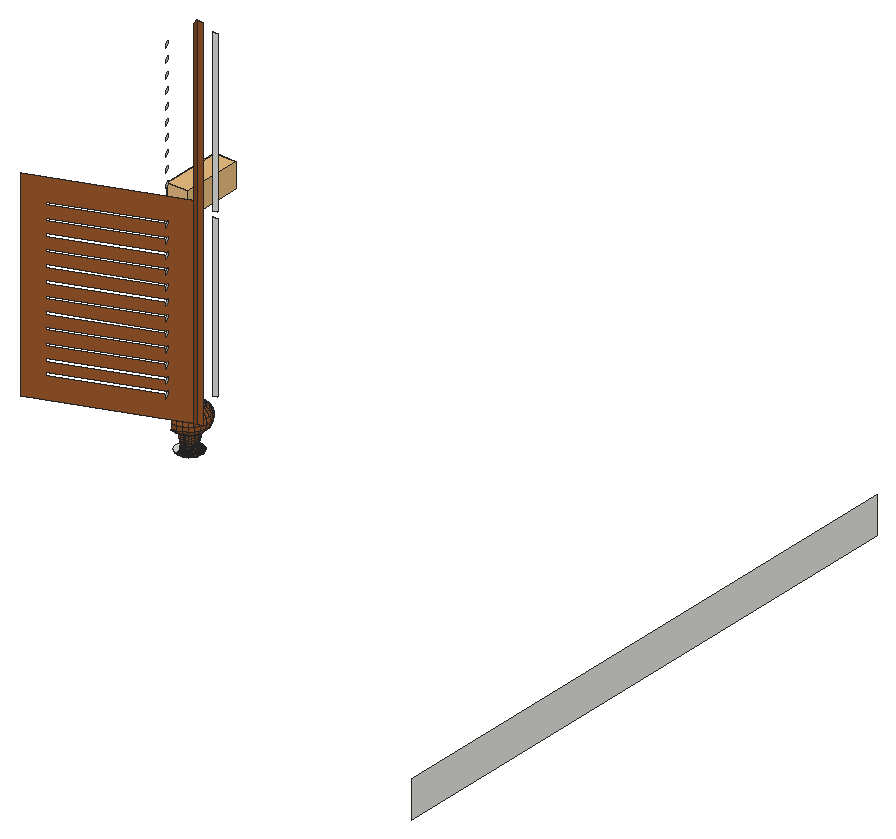
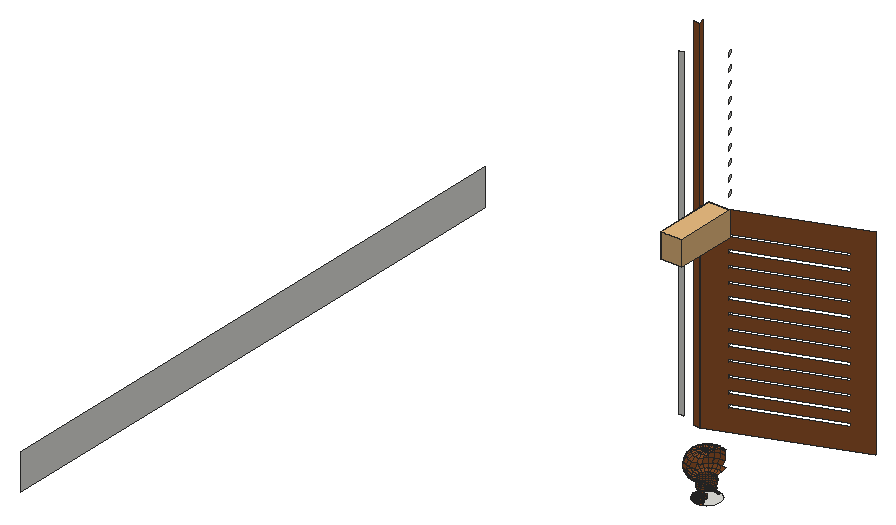
# SketchUp Ruby script. Lengths in inches.
U = 1.inch
M = Sketchup.active_model
def pt(a) = Geom::Point3d.new(a.map { |v| v * U })
def face(e, loops, mat)
  f = e.add_face(loops[0].map { |a| pt(a) })
  loops[1..].each { |l| e.add_face(l.map { |a| pt(a) }).erase! }
  f.material = f.back_material = mat if mat
  f
end
# faces: each face lists its corners as indices into pts; further lists are holes
def faces(e, pts, list, mat = nil) = list.each { |f| face(e, (f[0].is_a?(Array) ? f : [f]).map { |l| l.map { |i| pts[i] } }, mat) }
# xy, xz, yz: faces in a plane at the given z, y or x. An outline is a flat list of corners, or four numbers for a rectangle; further outlines are holes
def ring(l) = l.size == 4 ? [[l[0], l[1]], [l[2], l[1]], [l[2], l[3]], [l[0], l[3]]] : l.each_slice(2).to_a
def flat(e, list, mat, &to3) = list.each { |f| face(e, (f[0].is_a?(Array) ? f : [f]).map { |l| ring(l).map { |u, v| to3.(u, v) } }, mat) }
def xy(e, z, list, mat = nil) = flat(e, list, mat) { |x, y| [x, y, z] }
def xz(e, y, list, mat = nil) = flat(e, list, mat) { |x, z| [x, y, z] }
def yz(e, x, list, mat = nil) = flat(e, list, mat) { |y, z| [x, y, z] }
def lines(e, pts, list) = list.each { |a, b| e.add_line(pt(pts[a]), pt(pts[b])) }
# prism: a flat outline (further loops are holes) pulled along v
def prism(e, loops, v, mat = nil)
  f = face(e, loops, mat); d = Geom::Vector3d.new(v.map { |x| x * U })
  f.pushpull(f.normal.samedirection?(d) ? d.length : -d.length)
end
def box(e, o, s, mat = nil) = prism(e, [[o, [o[0] + s[0], o[1], o[2]], [o[0] + s[0], o[1] + s[1], o[2]], [o[0], o[1] + s[1], o[2]]]], [0, 0, s[2]], mat)
def at(x, y, z, deg = 0) = Geom::Transformation.translation(pt([x, y, z])) * Geom::Transformation.rotation(ORIGIN, Z_AXIS, deg.degrees)
def axes(o, x, y, z) = Geom::Transformation.new([*x, 0, *y, 0, *z, 0, *pt(o).to_a, 1])
def part(name) = M.definitions.add(name)
# library, detail: a bought-in or finely detailed component or shape, given as its bounding box
def library(name, o, s) = part(name).tap { |d| box(d.entities, o, s) }
def detail(e, o, s) = box(e.add_group.entities, o, s)
def put(e, d, t, mat = nil) = e.add_instance(d, t).tap { |i| i.material = mat if mat }
def group(e, t, mat = nil) = e.add_group.tap { |g| g.transformation = t; g.material = mat if mat }.entities
root = M.entities
M.materials.add("[Color M03]").color = [170, 170, 170]
M.materials.add("[Wood Cherry Original]").color = [152, 86, 42]
c1 = library("Group\#10",[0,0,0],[6.05,17.1,6.94])
xy(root,6,[[197.18,47.97,197.74,47.97,198.28,48.11,198.76,48.39,199.16,48.78,199.4375,49.26,199.59,49.8,199.59,50.36,199.44,50.9,199.17,51.38,198.77,51.78,198.29,52.06,197.75,52.21,197.19,52.21,196.65,52.07,196.17,51.79,195.77,51.4,195.49,50.91,195.35,50.375,195.34,49.82,195.49,49.28,195.76,48.79,196.16,48.4,196.64,48.11]])
xy(root,6,[[197.18,47.97,197.2,48.12,196.7,48.25,196.64,48.11],[197.18,47.97,197.74,47.97,197.72,48.12,197.2,48.12],[197.74,47.97,198.28,48.11,198.22,48.25,197.72,48.12],[198.28,48.11,198.76,48.39,198.67,48.51,198.22,48.25],[198.76,48.39,199.16,48.78,199.04,48.87,198.67,48.51],
  [199.16,48.78,199.4375,49.26,199.3,49.32,199.04,48.87],[199.4375,49.26,199.59,49.8,199.44,49.82,199.3,49.32],[199.59,49.8,199.59,50.36,199.4375,50.34,199.44,49.82],[199.4375,50.34,199.59,50.36,199.44,50.9,199.3,50.84],[199.3,50.84,199.44,50.9,199.17,51.38,199.05,51.29],
  [199.05,51.29,199.17,51.38,198.77,51.78,198.68,51.66],[198.68,51.66,198.77,51.78,198.29,52.06,198.23,51.92],[198.23,51.92,198.29,52.06,197.75,52.21,197.73,52.06],[196.71,51.93,197.21,52.06,197.19,52.21,196.65,52.07],[197.21,52.06,197.73,52.06,197.75,52.21,197.19,52.21]],"[Wood Cherry Original]")
xz(root,46.11,[[201.81,13.08,202.9,73.08]],"[Wood Cherry Original]")
xz(root,48.59,[[197.26,8.1,197.66,8.4]],"[Wood Cherry Original]")
xz(root,49.11,[[202.15,16.08,202.9,42.58],[202.15,43.58,202.9,70.08]])
xz(root,51.28,[[197.3125,6.79,197.63,6.94]],"[Wood Cherry Original]")
yz(root,198.66,[[49.93,6.79,50.24,6.94]],"[Wood Cherry Original]")
yz(root,198.96,[[49.88,8.1,50.28,8.4]],"[Wood Cherry Original]")
yz(root,274.48,[[0,0,96.25,6]])
p = [[196.76,48.39,6.03],[196.7,48.25,6],[197.2,48.12,6],[197.22,48.27,6.03],[197.72,48.12,6],[197.7,48.26,6.03],
  [198.22,48.25,6],[198.16,48.39,6.03],[198.67,48.51,6],[198.58,48.625,6.03],[196.81,48.52,6.08],[197.24,48.41,6.08],
  [197.68,48.4,6.08],[198.11,48.52,6.08],[198.49,48.74,6.08],[199.04,48.87,6],[198.92,48.96,6.03],[198.81,49.05,6.08],
  [199.3,49.32,6],[199.16,49.375,6.03],[199.03,49.43,6.08],[199.44,49.82,6],[199.29,49.84,6.03],[199.15,49.86,6.08],
  [199.29,50.32,6.03],[199.15,50.3,6.08],[199.4375,50.34,6],[199.17,50.78,6.03],[199.04,50.73,6.08],[199.3,50.84,6],
  [198.93,51.2,6.03],[198.82,51.11,6.08],[199.05,51.29,6],[198.59,51.54,6.03],[198.5,51.43,6.08],[198.68,51.66,6],
  [198.18,51.78,6.03],[198.12,51.65,6.08],[198.23,51.92,6],[197.25,51.77,6.08],[197.23,51.91,6.03],[196.77,51.79,6.03],
  [196.82,51.66,6.08],[197.71,51.91,6.03],[197.69,51.77,6.08],[197.21,52.06,6],[196.71,51.93,6],[197.73,52.06,6],
  [196.86,48.64,6.16],[197.26,48.54,6.16],[197.66,48.53,6.16],[198.06,48.64,6.16],[198.41,48.84,6.16],[198.7,49.13,6.16],
  [198.91,49.48,6.16],[199.02,49.875,6.16],[199.02,50.29,6.16],[198.91,50.68,6.16],[198.71,51.04,6.16],[198.42,51.33,6.16],
  [198.07,51.53,6.16],[197.27,51.64,6.16],[196.87,51.54,6.16],[197.68,51.64,6.16],[196.91,48.75,6.25],[197.27,48.65,6.25],
  [197.65,48.65,6.25],[198.02,48.74,6.25],[198.34,48.93,6.25],[198.61,49.2,6.25],[198.8,49.53,6.25],[198.9,49.89,6.25],
  [198.9,50.27,6.25],[198.81,50.64,6.25],[198.62,50.97,6.25],[198.35,51.23,6.25],[198.03,51.43,6.25],[197.28,51.53,6.25],
  [196.92,51.43,6.25],[197.66,51.52,6.25],[196.94,48.84,6.37],[197.28,48.75,6.37],[197.64,48.74,6.37],[197.98,48.83,6.37],
  [198.29,49.01,6.37],[198.54,49.26,6.37],[198.71,49.5625,6.37],[198.81,49.91,6.37],[198.81,50.26,6.37],[198.72,50.6,6.37],
  [198.54,50.91,6.37],[198.29,51.16,6.37],[197.99,51.34,6.37],[197.29,51.43,6.37],[196.95,51.34,6.37],[197.65,51.43,6.37],
  [196.97,48.91,6.5],[197.29,48.82,6.5],[197.63,48.82,6.5],[197.95,48.9,6.5],[198.24,49.07,6.5],[198.48,49.3,6.5],
  [198.65,49.59,6.5],[198.73,49.92,6.5],[198.73,50.25,6.5],[198.65,50.57,6.5],[198.48,50.86,6.5],[198.25,51.1,6.5],
  [197.96,51.27,6.5],[197.3,51.36,6.5],[196.98,51.27,6.5],[197.64,51.35,6.5],[196.99,48.95,6.64],[197.3,48.87,6.64],
  [197.62,48.87,6.64],[197.93,48.95,6.64],[196.71,49.12,6.64],[196.68,49.08,6.5],[198.21,49.11,6.64],[198.4375,49.34,6.64],
  [198.6,49.61,6.64],[198.68,49.92,6.64],[198.68,50.24,6.64],[198.6,50.55,6.64],[198.44,50.83,6.64],[198.22,51.06,6.64],
  [197,51.22,6.64],[196.69,51.1,6.5],[196.72,51.0625,6.64],[197.94,51.22,6.64],[197.31,51.3,6.64],[197.63,51.3,6.64],
  [197,48.98,6.79],[197.3,48.9,6.79],[197.62,48.9,6.79],[197.92,48.98,6.79],[196.73,49.14,6.79],[198.19,49.13,6.79],
  [198.42,49.35,6.79],[198.57,49.62,6.79],[198.66,49.93,6.79],[198.66,50.24,6.79],[198.58,50.54,6.79],[198.42,50.82,6.79],
  [198.2,51.04,6.79],[197.01,51.2,6.79],[196.74,51.04,6.79],[197.93,51.2,6.79],[197.3125,51.28,6.79],[197.63,51.28,6.79],
  [197,48.98,6.94],[197.3,48.9,6.94],[197.62,48.89,6.94],[197.92,48.97,6.94],[196.73,49.14,6.94],[198.19,49.13,6.94],
  [198.42,49.35,6.94],[198.57,49.62,6.94],[198.66,49.93,6.94],[198.66,50.24,6.94],[198.58,50.54,6.94],[198.42,50.82,6.94],
  [198.2,51.04,6.94],[197.01,51.2,6.94],[196.74,51.04,6.94],[197.93,51.2,6.94],[197.3125,51.28,6.94],[197.63,51.28,6.94],
  [196.99,48.95,7.09],[197.3,48.87,7.09],[197.62,48.87,7.09],[197.93,48.95,7.09],[196.71,49.12,7.09],[198.21,49.11,7.09],
  [198.4375,49.34,7.09],[198.6,49.61,7.09],[198.68,49.92,7.09],[198.68,50.24,7.09],[198.6,50.55,7.09],[198.44,50.83,7.09],
  [198.22,51.06,7.09],[197,51.22,7.09],[196.72,51.06,7.09],[197.94,51.22,7.09],[197.31,51.31,7.09],[197.63,51.3,7.09],
  [196.97,48.91,7.23],[197.29,48.82,7.23],[197.63,48.82,7.23],[197.95,48.9,7.23],[196.68,49.07,7.23],[198.24,49.07,7.23],
  [198.48,49.3,7.23],[198.65,49.59,7.23],[198.73,49.92,7.23],[198.74,50.25,7.23],[198.65,50.57,7.23],[198.48,50.86,7.23],
  [198.25,51.1,7.23],[196.98,51.27,7.23],[196.69,51.11,7.23],[197.96,51.27,7.23],[197.3,51.36,7.23],[197.64,51.36,7.23],
  [196.93,48.8,7.51],[197.28,48.71,7.51],[197.64,48.71,7.51],[197.99,48.8,7.51],[198.31,48.98,7.51],[198.57,49.24,7.51],
  [198.75,49.55,7.51],[198.84,49.9,7.51],[198.85,50.26,7.51],[198.75,50.61,7.51],[198.57,50.93,7.51],[198.32,51.1875,7.51],
  [198,51.37,7.51],[197.29,51.47,7.51],[196.9375,51.375,7.51],[197.65,51.47,7.51],[196.9,48.73,7.8],[197.27,48.63,7.8],
  [197.65,48.63,7.8],[198.02,48.73,7.8],[198.35,48.92,7.8],[198.625,49.1875,7.8],[198.82,49.52,7.8],[198.92,49.89,7.8],
  [198.92,50.27,7.8],[198.82,50.64,7.8],[198.63,50.98,7.8],[198.36,51.25,7.8],[198.03,51.44,7.8],[197.28,51.54,7.8],
  [196.91,51.45,7.8],[197.66,51.54,7.8],[196.88,48.7,8.1],[197.26,48.59,8.1],[197.66,48.59,8.1],[198.04,48.69,8.1],
  [198.38,48.89,8.1],[198.66,49.16,8.1],[198.86,49.5,8.1],[198.96,49.88,8.1],[198.96,50.28,8.1],[198.86,50.66,8.1],
  [198.66,51,8.1],[198.39,51.28,8.1],[198.05,51.48,8.1],[197.27,51.58,8.1],[196.89,51.48,8.1],[197.67,51.58,8.1],
  [196.88,48.69,8.4],[197.26,48.59,8.4],[197.66,48.59,8.4],[198.04,48.69,8.4],[198.38,48.89,8.4],[198.66,49.16,8.4],
  [198.86,49.5,8.4],[198.96,49.88,8.4],[198.96,50.28,8.4],[198.86,50.66,8.4],[198.67,51,8.4],[198.39,51.28,8.4],
  [198.05,51.48,8.4],[197.27,51.59,8.4],[196.89,51.48,8.4],[197.67,51.58,8.4],[196.9,48.73,8.7],[197.27,48.625,8.7],
  [197.65,48.62,8.7],[198.03,48.72,8.7],[198.36,48.91,8.7],[198.63,49.18,8.7],[198.83,49.52,8.7],[198.93,49.89,8.7],
  [198.93,50.27,8.7],[198.83,50.65,8.7],[198.64,50.98,8.7],[198.37,51.25,8.7],[198.04,51.45,8.7],[197.66,51.55,8.7],
  [197.28,51.55,8.7],[196.91,51.45,8.7],[196.92,48.79,8.99],[197.28,48.69,8.99],[197.64,48.69,8.99],[198,48.79,8.99],
  [198.32,48.97,8.99],[198.58,49.23,8.99],[198.76,49.54,8.99],[198.86,49.9,8.99],[198.86,50.27,8.99],[198.77,50.62,8.99],
  [198.58,50.9375,8.99],[198.33,51.2,8.99],[198.01,51.38,8.99],[197.29,51.48,8.99],[196.93,51.39,8.99],[197.65,51.48,8.99],
  [196.65,48.14,9.21],[197.18,48,9.21],[197.73,48,9.21],[198.26,48.14,9.21],[198.74,48.41,9.21],[199.13,48.8,9.21],
  [199.41,49.27,9.21],[199.55,49.8,9.21],[199.56,50.35,9.21],[199.42,50.89,9.21],[199.14,51.36,9.21],[198.76,51.75,9.21],
  [198.28,52.03,9.21],[197.2,52.18,9.21],[196.67,52.04,9.21],[197.75,52.18,9.21],[196.43,47.61,9.66],[197.1,47.42,9.66],
  [197.81,47.42,9.66],[198.48,47.6,9.66],[199.09,47.95,9.66],[199.59,48.44,9.66],[199.94,49.05,9.66],[200.13,49.73,9.66],
  [200.13,50.43,9.66],[199.95,51.11,9.66],[199.6,51.71,9.66],[199.11,52.21,9.66],[198.5,52.57,9.66],[197.125,52.75,9.66],
  [196.45,52.57,9.66],[197.83,52.75,9.66],[197.05,47.05,10.28],[197.85,47.04,10.28],[198.63,47.25,10.28],[199.32,47.65,10.28],
  [199.89,48.21,10.28],[200.29,48.9,10.28],[200.51,49.68,10.28],[200.51,50.48,10.28],[200.3,51.25,10.28],[199.91,51.94,10.28],
  [199.34,52.51,10.28],[198.65,52.92,10.28],[197.88,53.125,10.28],[197.08,53.13,10.28],[197.04,46.92,11],[197.87,46.91,11],
  [198.68,47.125,11],[199.4,47.54,11],[200,48.13,11],[200.42,48.85,11],[200.64,49.66,11],[200.64,50.49,11],
  [200.43,51.3,11],[200.01,52.03,11],[199.42,52.62,11],[198.7,53.04,11],[197.05,47.05,11.72],[197.85,47.04,11.72],
  [198.63,47.25,11.72],[199.32,47.65,11.72],[199.89,48.21,11.72],[200.29,48.9,11.72],[200.51,49.68,11.72],[200.51,50.48,11.72],
  [200.3,51.25,11.72],[199.91,51.94,11.72],[199.34,52.51,11.72],[198.65,52.92,11.72],[197.1,47.42,12.34],[197.81,47.42,12.34],
  [198.48,47.6,12.34],[199.09,47.95,12.34],[199.59,48.44,12.34],[199.94,49.05,12.34],[200.13,49.73,12.34],[200.13,50.43,12.34],
  [199.95,51.11,12.34],[199.6,51.71,12.34],[199.11,52.21,12.34],[198.5,52.57,12.34],[197.88,53.125,11.72],[197.83,52.75,12.34],
  [197.08,53.13,11.72],[197.125,52.75,12.34],[196.65,48.14,12.79],[196.43,47.61,12.34],[197.18,48,12.79],[197.73,48,12.79],
  [198.26,48.14,12.79],[198.74,48.41,12.79],[199.13,48.8,12.79],[199.41,49.27,12.79],[199.55,49.8,12.79],[199.56,50.35,12.79],
  [199.42,50.89,12.79],[199.14,51.36,12.79],[198.76,51.75,12.79],[198.28,52.03,12.79],[197.2,52.18,12.79],[196.45,52.57,12.34],
  [196.67,52.04,12.79],[197.75,52.18,12.79],[197.47,50.09,12.67],[197.21,49.47,12.97],[197.375,49.42,12.97],[197.55,49.42,12.97],
  [197.72,49.47,12.97],[197.05,49.56,12.97],[197.87,49.55,12.97],[196.93,49.68,12.97],[198,49.68,12.97],[196.84,49.83,12.97],
  [198.08,49.83,12.97],[196.8,50,12.97],[198.13,50,12.97],[196.8,50.18,12.97],[198.13,50.17,12.97],[196.85,50.35,12.97],
  [196.93,50.5,12.97],[197.06,50.62,12.97],[197.21,50.71,12.97],[197.38,50.75,12.97],[197.56,50.75,12.97],[197.72,50.71,12.97],
  [197.875,50.62,12.97],[198,50.49,12.97],[198.09,50.34,12.97],[196.92,48.79,13.01],[197.28,48.69,13.01],[197.64,48.69,13.01],
  [198,48.79,13.01],[198.32,48.97,13.01],[198.58,49.23,13.01],[198.76,49.54,13.01],[198.86,49.9,13.01],[198.86,50.27,13.01],
  [198.77,50.62,13.01],[198.58,50.9375,13.01],[198.33,51.2,13.01],[198.01,51.38,13.01],[197.29,51.48,13.01],[196.93,51.39,13.01],
  [197.65,51.48,13.01],[196.61,48.98,13.01],[196.61,51.21,13.01],[201.81,46.11,14.08],[201.81,46.11,13.08],[179.45,37.53,13.08],
  [179.45,37.53,46.26],[201.81,46.11,46.26],[201.81,46.11,43.08],[201.81,46.11,42.08],[201.81,46.11,28.58],[201.81,46.11,27.58],
  [198.23,44.74,16.73],[198.23,44.74,17.26],[182.72,38.79,17.26],[182.72,38.79,16.73],[182.72,38.79,42.58],[182.72,38.79,42.08],
  [198.23,44.74,42.08],[198.23,44.74,42.58],[182.72,38.79,40.25],[182.72,38.79,39.75],[198.23,44.74,39.75],[198.23,44.74,40.25],
  [182.72,38.79,37.93],[182.72,38.79,37.43],[198.23,44.74,37.43],[198.23,44.74,37.93],[182.72,38.79,35.6],[182.72,38.79,35.1],
  [198.23,44.74,35.1],[198.23,44.74,35.6],[182.72,38.79,33.28],[182.72,38.79,32.78],[198.23,44.74,32.78],[198.23,44.74,33.28],
  [182.72,38.79,30.95],[182.72,38.79,30.45],[198.23,44.74,30.45],[198.23,44.74,30.95],[182.72,38.79,28.625],[182.72,38.79,28.125],
  [198.23,44.74,28.125],[198.23,44.74,28.625],[182.72,38.79,26.3],[182.72,38.79,25.8],[198.23,44.74,25.8],[198.23,44.74,26.3],
  [182.72,38.79,23.98],[182.72,38.79,23.48],[198.23,44.74,23.48],[198.23,44.74,23.98],[198.23,44.74,18.83],[198.23,44.74,19.33],
  [182.72,38.79,19.33],[182.72,38.79,18.83],[182.72,38.79,21.65],[182.72,38.79,21.15],[198.23,44.74,21.15],[198.23,44.74,21.65],
  [202.17,45.18,13.08],[201.81,46.11,56.58],[201.81,46.11,57.58],[201.81,46.11,72.08],[201.81,46.11,73.08],[202.17,45.18,73.08],
  [198.59,43.81,16.73],[198.59,43.81,17.26],[198.59,43.81,18.83],[198.59,43.81,19.33],[198.59,43.81,21.15],[198.59,43.81,21.65],
  [198.59,43.81,23.48],[198.59,43.81,23.98],[198.59,43.81,25.8],[198.59,43.81,26.3],[198.59,43.81,28.125],[198.59,43.81,28.625],
  [198.59,43.81,30.45],[198.59,43.81,30.95],[198.59,43.81,32.78],[198.59,43.81,33.28],[198.59,43.81,35.1],[198.59,43.81,35.6],
  [198.59,43.81,37.43],[198.59,43.81,37.93],[198.59,43.81,39.75],[198.59,43.81,40.25],[198.59,43.81,42.08],[198.59,43.81,42.58],
  [198.59,43.81,47.97],[198.59,43.81,48.47],[198.23,44.74,48.47],[198.23,44.74,47.97],[198.59,43.81,50.29],[198.59,43.81,50.79],
  [198.23,44.74,50.79],[198.23,44.74,50.29],[198.59,43.81,52.62],[198.59,43.81,53.12],[198.23,44.74,53.12],[198.23,44.74,52.62],
  [198.59,43.81,54.94],[198.59,43.81,55.44],[198.23,44.74,55.44],[198.23,44.74,54.94],[198.59,43.81,57.27],[198.59,43.81,57.77],
  [198.23,44.74,57.77],[198.23,44.74,57.27],[198.59,43.81,59.59],[198.59,43.81,60.09],[198.23,44.74,60.09],[198.23,44.74,59.59],
  [198.59,43.81,61.92],[198.59,43.81,62.42],[198.23,44.74,62.42],[198.23,44.74,61.92],[198.59,43.81,64.24],[198.59,43.81,64.74],
  [198.23,44.74,64.74],[198.23,44.74,64.24],[198.59,43.81,66.57],[198.59,43.81,67.07],[198.23,44.74,67.07],[198.23,44.74,66.57],
  [198.59,43.81,68.89],[198.59,43.81,69.39],[198.23,44.74,69.39],[198.23,44.74,68.89]]
faces(root,p,[[0,1,2,3],[3,2,4,5],[5,4,6,7],[7,6,8,9],[10,0,3,11],[11,3,5,12],[12,5,7,13],[13,7,9,14],
  [9,8,15,16],[14,9,16,17],[16,15,18,19],[17,16,19,20],[19,18,21,22],[20,19,22,23],[23,22,24,25],[22,21,26,24],
  [25,24,27,28],[24,26,29,27],[28,27,30,31],[27,29,32,30],[31,30,33,34],[30,32,35,33],[34,33,36,37],[33,35,38,36],
  [39,40,41,42],[37,36,43,44],[40,45,46,41],[44,43,40,39],[36,38,47,43],[43,47,45,40],[48,10,11,49],[49,11,12,50],
  [50,12,13,51],[51,13,14,52],[52,14,17,53],[53,17,20,54],[54,20,23,55],[55,23,25,56],[56,25,28,57],[57,28,31,58],
  [58,31,34,59],[59,34,37,60],[61,39,42,62],[60,37,44,63],[63,44,39,61],[64,48,49,65],[65,49,50,66],[66,50,51,67],
  [67,51,52,68],[68,52,53,69],[69,53,54,70],[70,54,55,71],[71,55,56,72],[72,56,57,73],[73,57,58,74],[74,58,59,75],
  [75,59,60,76],[77,61,62,78],[76,60,63,79],[79,63,61,77],[80,64,65,81],[81,65,66,82],[82,66,67,83],[83,67,68,84],
  [84,68,69,85],[85,69,70,86],[86,70,71,87],[87,71,72,88],[88,72,73,89],[89,73,74,90],[90,74,75,91],[91,75,76,92],
  [93,77,78,94],[92,76,79,95],[95,79,77,93],[96,80,81,97],[97,81,82,98],[98,82,83,99],[99,83,84,100],[100,84,85,101],
  [101,85,86,102],[102,86,87,103],[103,87,88,104],[104,88,89,105],[105,89,90,106],[106,90,91,107],[107,91,92,108],[109,93,94,110],
  [108,92,95,111],[111,95,93,109],[112,96,97,113],[113,97,98,114],[114,98,99,115],[116,117,96,112],[115,99,100,118],[118,100,101,119],
  [119,101,102,120],[120,102,103,121],[121,103,104,122],[122,104,105,123],[123,105,106,124],[124,106,107,125],[126,110,127,128],[125,107,108,129],
  [130,109,110,126],[129,108,111,131],[131,111,109,130],[132,112,113,133],[133,113,114,134],[134,114,115,135],[136,116,112,132],[135,115,118,137],
  [137,118,119,138],[138,119,120,139],[139,120,121,140],[140,121,122,141],[141,122,123,142],[142,123,124,143],[143,124,125,144],[145,126,128,146],
  [144,125,129,147],[148,130,126,145],[147,129,131,149],[149,131,130,148],[150,132,133,151],[151,133,134,152],[152,134,135,153],[154,136,132,150],
  [153,135,137,155],[155,137,138,156],[156,138,139,157],[157,139,140,158],[159,141,142,160],[160,142,143,161],[161,143,144,162],[163,145,146,164],
  [162,144,147,165],[166,148,145,163],[165,147,149,167],[168,150,151,169],[169,151,152,170],[170,152,153,171],[172,154,150,168],[171,153,155,173],
  [173,155,156,174],[174,156,157,175],[175,157,158,176],[176,158,159,177],[177,159,160,178],[178,160,161,179],[179,161,162,180],[181,163,164,182],
  [180,162,165,183],[184,166,163,181],[183,165,167,185],[185,167,166,184],[186,168,169,187],[187,169,170,188],[188,170,171,189],[190,172,168,186],
  [189,171,173,191],[191,173,174,192],[192,174,175,193],[193,175,176,194],[194,176,177,195],[195,177,178,196],[196,178,179,197],[197,179,180,198],
  [199,181,182,200],[198,180,183,201],[202,184,181,199],[201,183,185,203],[203,185,184,202],[204,186,187,205],[205,187,188,206],[206,188,189,207],
  [207,189,191,208],[208,191,192,209],[209,192,193,210],[210,193,194,211],[211,194,195,212],[212,195,196,213],[213,196,197,214],[214,197,198,215],
  [215,198,201,216],[217,202,199,218],[216,201,203,219],[219,203,202,217],[220,204,205,221],[221,205,206,222],[222,206,207,223],[223,207,208,224],
  [224,208,209,225],[225,209,210,226],[226,210,211,227],[227,211,212,228],[228,212,213,229],[229,213,214,230],[230,214,215,231],[231,215,216,232],
  [233,217,218,234],[232,216,219,235],[235,219,217,233],[236,220,221,237],[237,221,222,238],[238,222,223,239],[239,223,224,240],[240,224,225,241],
  [241,225,226,242],[242,226,227,243],[243,227,228,244],[244,228,229,245],[245,229,230,246],[246,230,231,247],[247,231,232,248],[249,233,234,250],
  [248,232,235,251],[251,235,233,249],[252,236,237,253],[254,238,239,255],[255,239,240,256],[256,240,241,257],[257,241,242,258],[258,242,243,259],
  [260,244,245,261],[261,245,246,262],[262,246,247,263],[263,247,248,264],[265,249,250,266],[264,248,251,267],[267,251,249,265],[268,252,253,269],
  [269,253,254,270],[270,254,255,271],[271,255,256,272],[272,256,257,273],[273,257,258,274],[274,258,259,275],[275,259,260,276],[276,260,261,277],
  [277,261,262,278],[278,262,263,279],[279,263,264,280],[280,264,267,281],[282,265,266,283],[281,267,265,282],[284,268,269,285],[285,269,270,286],
  [286,270,271,287],[287,271,272,288],[288,272,273,289],[289,273,274,290],[290,274,275,291],[291,275,276,292],[292,276,277,293],[293,277,278,294],
  [294,278,279,295],[295,279,280,296],[297,282,283,298],[296,280,281,299],[299,281,282,297],[300,284,285,301],[301,285,286,302],[302,286,287,303],
  [303,287,288,304],[304,288,289,305],[305,289,290,306],[306,290,291,307],[307,291,292,308],[308,292,293,309],[309,293,294,310],[310,294,295,311],
  [311,295,296,312],[313,297,298,314],[312,296,299,315],[315,299,297,313],[316,300,301,317],[317,301,302,318],[318,302,303,319],[319,303,304,320],
  [320,304,305,321],[321,305,306,322],[322,306,307,323],[323,307,308,324],[324,308,309,325],[325,309,310,326],[326,310,311,327],[327,311,312,328],
  [329,313,314,330],[328,312,315,331],[331,315,313,329],[332,317,318,333],[333,318,319,334],[334,319,320,335],[335,320,321,336],[336,321,322,337],
  [337,322,323,338],[338,323,324,339],[339,324,325,340],[340,325,326,341],[341,326,327,342],[342,327,328,343],[343,328,331,344],[344,331,329,345],
  [346,332,333,347],[347,333,334,348],[348,334,335,349],[349,335,336,350],[350,336,337,351],[351,337,338,352],[352,338,339,353],[353,339,340,354],
  [354,340,341,355],[355,341,342,356],[356,342,343,357],[358,346,347,359],[359,347,348,360],[360,348,349,361],[361,349,350,362],[362,350,351,363],
  [363,351,352,364],[364,352,353,365],[365,353,354,366],[366,354,355,367],[367,355,356,368],[368,356,357,369],[370,358,359,371],[371,359,360,372],
  [372,360,361,373],[373,361,362,374],[374,362,363,375],[375,363,364,376],[376,364,365,377],[377,365,366,378],[378,366,367,379],[379,367,368,380],
  [380,368,369,381],[381,369,382,383],[383,382,384,385],[386,387,370,388],[388,370,371,389],[389,371,372,390],[390,372,373,391],[391,373,374,392],
  [392,374,375,393],[393,375,376,394],[394,376,377,395],[395,377,378,396],[396,378,379,397],[397,379,380,398],[398,380,381,399],[400,385,401,402],
  [399,381,383,403],[403,383,385,400],[404,405,406],[404,406,407],[404,407,408],[404,409,405],[404,408,410],[404,411,409],
  [404,410,412],[404,413,411],[404,412,414],[404,415,413],[404,414,416],[404,417,415],[404,416,418],[404,419,417],
  [404,420,419],[404,421,420],[404,422,421],[404,423,422],[404,424,423],[404,425,424],[404,426,425],[404,427,426],
  [404,428,427],[404,418,428],[429,386,388,430],[430,388,389,431],[431,389,390,432],[432,390,391,433],[433,391,392,434],[434,392,393,435],
  [435,393,394,436],[436,394,395,437],[437,395,396,438],[438,396,397,439],[439,397,398,440],[440,398,399,441],[442,400,402,443],[441,399,403,444],
  [444,403,400,442],[405,429,430,406],[406,430,431,407],[407,431,432,408],[409,445,429,405],[408,432,433,410],[410,433,434,412],[412,434,435,414],
  [414,435,436,416],[416,436,437,418],[418,437,438,428],[428,438,439,427],[427,439,440,426],[422,443,446,421],[426,440,441,425],[423,442,443,422],
  [425,441,444,424],[424,444,442,423],[[447,448,449,450,451,452,453,454,455],[456,457,458,459],[460,461,462,463],[464,465,466,467],[468,469,470,471],[472,473,474,475],[476,477,478,479],[480,481,482,483],[484,485,486,487],[488,489,490,491],[492,493,494,495],[496,497,498,499],[500,501,502,503]],[504,448,447,455,454,453,452,451,505,506,507,508,509]],"[Wood Cherry Original]")
faces(root,p,[[510,511,457,456],[512,513,497,496],[514,515,503,502],[516,517,495,494],[518,519,491,490],[520,521,487,486],[522,523,483,482],[524,525,479,478],
  [526,527,475,474],[528,529,471,470],[530,531,467,466],[532,533,463,462],[534,535,536,537],[538,539,540,541],[542,543,544,545],[546,547,548,549],
  [550,551,552,553],[554,555,556,557],[558,559,560,561],[562,563,564,565],[566,567,568,569],[570,571,572,573]])
put(root,c1,axes([196.82,46.11,43.08],[0.5865,0,0],[0,0.5865,0],[0,0,0.5865]),"[Color M03]")
